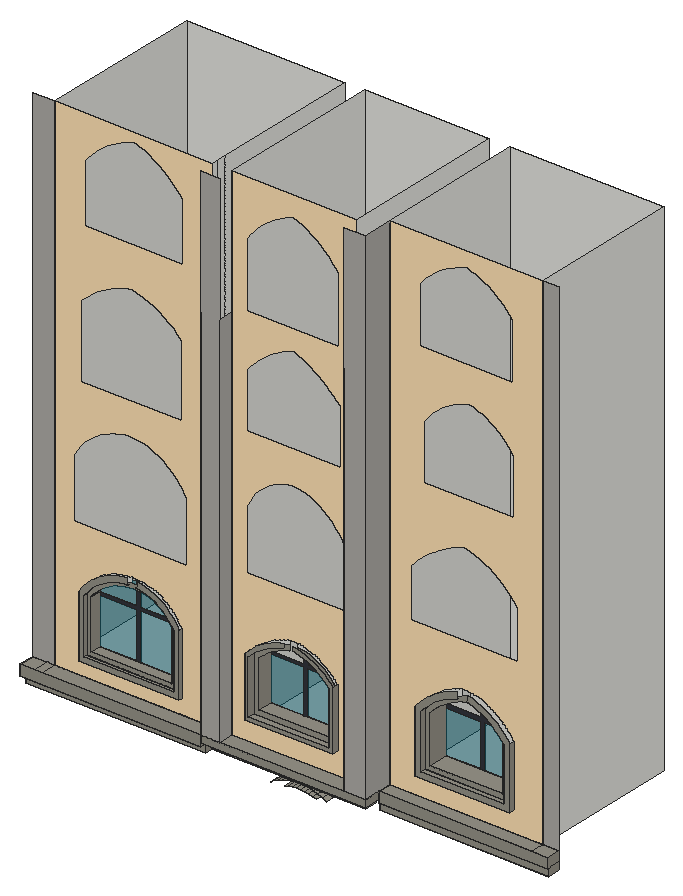
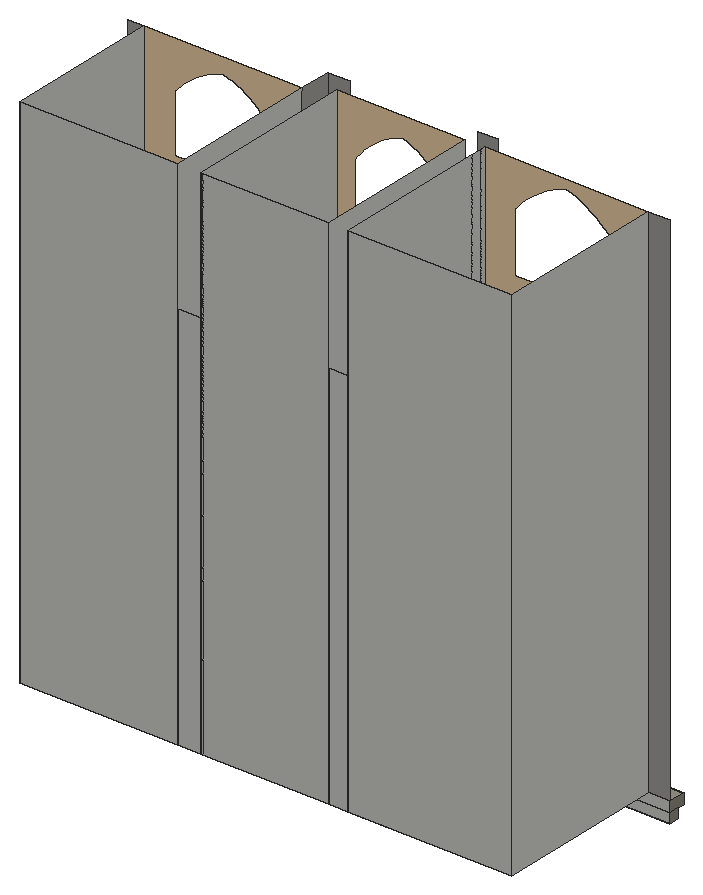
# SketchUp Ruby script. Lengths in inches.
U = 1.inch
M = Sketchup.active_model
def pt(a) = Geom::Point3d.new(a.map { |v| v * U })
def face(e, loops, mat)
  f = e.add_face(loops[0].map { |a| pt(a) })
  loops[1..].each { |l| e.add_face(l.map { |a| pt(a) }).erase! }
  f.material = f.back_material = mat if mat
  f
end
# faces: each face lists its corners as indices into pts; further lists are holes
def faces(e, pts, list, mat = nil) = list.each { |f| face(e, (f[0].is_a?(Array) ? f : [f]).map { |l| l.map { |i| pts[i] } }, mat) }
# xy, xz, yz: faces in a plane at the given z, y or x. An outline is a flat list of corners, or four numbers for a rectangle; further outlines are holes
def ring(l) = l.size == 4 ? [[l[0], l[1]], [l[2], l[1]], [l[2], l[3]], [l[0], l[3]]] : l.each_slice(2).to_a
def flat(e, list, mat, &to3) = list.each { |f| face(e, (f[0].is_a?(Array) ? f : [f]).map { |l| ring(l).map { |u, v| to3.(u, v) } }, mat) }
def xy(e, z, list, mat = nil) = flat(e, list, mat) { |x, y| [x, y, z] }
def xz(e, y, list, mat = nil) = flat(e, list, mat) { |x, z| [x, y, z] }
def yz(e, x, list, mat = nil) = flat(e, list, mat) { |y, z| [x, y, z] }
def lines(e, pts, list) = list.each { |a, b| e.add_line(pt(pts[a]), pt(pts[b])) }
# prism: a flat outline (further loops are holes) pulled along v
def prism(e, loops, v, mat = nil)
  f = face(e, loops, mat); d = Geom::Vector3d.new(v.map { |x| x * U })
  f.pushpull(f.normal.samedirection?(d) ? d.length : -d.length)
end
def box(e, o, s, mat = nil) = prism(e, [[o, [o[0] + s[0], o[1], o[2]], [o[0] + s[0], o[1] + s[1], o[2]], [o[0], o[1] + s[1], o[2]]]], [0, 0, s[2]], mat)
def at(x, y, z, deg = 0) = Geom::Transformation.translation(pt([x, y, z])) * Geom::Transformation.rotation(ORIGIN, Z_AXIS, deg.degrees)
def axes(o, x, y, z) = Geom::Transformation.new([*x, 0, *y, 0, *z, 0, *pt(o).to_a, 1])
def part(name) = M.definitions.add(name)
# library, detail: a bought-in or finely detailed component or shape, given as its bounding box
def library(name, o, s) = part(name).tap { |d| box(d.entities, o, s) }
def detail(e, o, s) = box(e.add_group.entities, o, s)
def put(e, d, t, mat = nil) = e.add_instance(d, t).tap { |i| i.material = mat if mat }
def group(e, t, mat = nil) = e.add_group.tap { |g| g.transformation = t; g.material = mat if mat }.entities
root = M.entities
M.materials.add("[Formica Beige]").color = [255, 225, 180]
M.materials.add("[Formica Graystone]").color = [149, 146, 135]
M.materials.add("[Formica Laminate Dark]").color = [50, 53, 60]
M.materials.add("[Terrazzo Tile Light]").color = [173, 171, 166]
M.materials.add("[Translucent Glass Tinted]").color = [4, 106, 127]
M.materials["[Translucent Glass Tinted]"].alpha = 0.48
xy(root,162.44,[[10.25,135.29,181.54,144.04]],"[Formica Graystone]")
xy(root,164.1875,[[338.35,146.55,499.12,158.3]],"[Formica Graystone]")
xy(root,167.08,[[186.17,137.18,186.17,148.61,199.67,148.61,199.67,158.3,317.75,158.3,317.75,148.61,332.68,148.61,332.68,137.18]],"[Formica Graystone]")
xy(root,171.09,[[10.25,135.29,181.54,144.04]])
xy(root,171.09,[[10.25,128.91,181.54,135.29]],"[Formica Graystone]")
xy(root,171.14,[[338.35,146.55,499.12,158.3]])
xy(root,171.14,[[338.35,145.11,499.12,146.55]],"[Formica Graystone]")
xy(root,174.01,[[186.17,137.18,186.17,148.61,199.67,148.61,199.67,158.3,317.75,158.3,317.75,148.61,332.68,148.61,332.68,137.18]])
xy(root,174.01,[[181.54,128.91,338.35,137.18],[181.54,137.18,186.17,148.61],[332.68,137.18,338.35,148.61]],"[Formica Graystone]")
xy(root,180.875,[[181.54,128.91,199.67,301.14],[317.75,128.91,338.35,158.3],[30.78,144.04,181.54,301.14],[199.67,144.04,317.75,158.3],[199.67,158.3,317.75,301.14],
  [317.75,158.3,338.35,301.14],[338.35,158.3,483.98,301.14]])
xy(root,180.875,[[10.25,128.91,24.51,144.04],[24.51,128.91,30.78,144.04],[30.78,128.91,181.54,144.04],[199.67,128.91,317.75,144.04],[338.35,145.11,483.98,158.3],
  [483.98,145.11,499.12,158.3]],"[Formica Graystone]")
xy(root,194.77,[[56.17,140.72,151.73,144.04]],"[Formica Graystone]")
xy(root,200.03,[[61.43,140.72,146.48,144.04]],"[Formica Graystone]")
xy(root,200.28,[[366.17,152.99,456.05,158.3]],"[Formica Graystone]")
xy(root,202.4375,[[216.67,137.35,300.3,144.04]],"[Formica Graystone]")
xy(root,203.83,[[65.22,144.04,142.68,154.66]],"[Formica Graystone]")
xy(root,205.7,[[371.6,152.99,450.625,158.3]],"[Formica Graystone]")
xy(root,206.125,[[220.36,137.35,296.61,144.04]],"[Formica Graystone]")
xy(root,210.3,[[376.19,158.3,446.03,177.43]],"[Formica Graystone]")
xy(root,210.91,[[225.15,144.04,291.83,158.22]],"[Formica Graystone]")
xz(root,128.91,[[10.25,171.09,181.54,180.875],[181.54,174.01,338.35,180.875]],"[Formica Graystone]")
xz(root,128.91,[[181.54,180.875,199.67,660.875],[317.75,180.875,338.35,660.875]],"[Terrazzo Tile Light]")
xz(root,135.29,[[10.25,162.44,181.54,171.09]],"[Formica Graystone]")
xz(root,137.18,[[186.17,167.08,332.68,174.01]],"[Formica Graystone]")
xz(root,137.35,[[216.67,202.4375,300.3,202.4375,300.3,258.75,297.68,261.875,294.86,264.8125,291.84,267.55,288.64,270.08,285.28,272.37,281.76,274.43,278.11,276.24,274.35,277.8,270.48,279.1,266.54,280.12,262.53,280.87,262.53,277.12,265.73,276.52,269.43,275.56,273.06,274.34,276.59,272.88,280.01,271.19,283.3,269.25,286.46,267.1,289.46,264.73,292.29,262.17,294.9375,259.41,296.61,257.41,296.61,206.125,220.36,206.125,220.36,257.22,222.06,258.93,224.9,261.5,227.88,263.91,230.98,266.16,234.2,268.25,237.52,270.16,240.9375,271.89,244.44,273.4375,248.03,274.8,251.68,275.97,254.54,276.72,254.54,280.53,250.64,279.51,246.81,278.28,243.04,276.85,239.36,275.22,235.76,273.4,232.27,271.4,228.89,269.21,225.63,266.84,222.51,264.3,219.52,261.6,216.67,258.75]],"[Formica Graystone]")
xz(root,140.72,[[56.17,194.77,151.73,194.77,151.73,253.84,149.35,258.08,146.5625,262.07,143.4,265.78,139.9,269.16,136.08,272.18,131.99,274.82,127.66,277.06,123.14,278.86,118.46,280.21,113.67,281.1,112.68,281.1875,112.68,276.05,111.06,276.05,112.96,275.88,117.24,275.09,121.43,273.875,125.48,272.26,129.35,270.27,133.02,267.9,136.43,265.2,139.57,262.17,142.4,258.86,144.89,255.28,146.48,252.46,146.48,200.03,61.43,200.03,61.43,252.15,63.1,254.5,65.9,257.84,68.95,260.96,72.23,263.83,75.73,266.4375,79.42,268.77,83.27,270.8,87.28,272.53,91.4,273.95,95.625,275.04,99.92,275.8,104.21,276.22,102.59,276.14,102.33,281.32,99.21,281.01,94.51,280.18,89.89,278.99,85.38,277.44,81,275.55,76.78,273.32,72.75,270.78,68.93,267.92,65.34,264.78,62,261.375,58.9375,257.72,56.17,253.84]],"[Formica Graystone]")
xz(root,144.04,[[10.25,162.44,181.54,171.09],[10.25,171.09,181.54,180.875],[56.17,194.77,56.17,253.84,58.9375,257.72,62,261.375,65.34,264.78,68.93,267.92,72.75,270.78,76.78,273.32,81,275.55,85.38,277.44,89.89,278.99,94.51,280.18,99.21,281.01,103.95,281.47,104.21,276.22,99.92,275.8,95.625,275.04,91.4,273.95,87.28,272.53,83.27,270.8,79.42,268.77,75.73,266.4375,72.23,263.83,68.95,260.96,65.9,257.84,63.1,254.5,61.43,252.15,61.43,200.03,146.48,200.03,146.48,252.46,144.89,255.28,142.4,258.86,139.57,262.17,136.43,265.2,133.02,267.9,129.35,270.27,125.48,272.26,121.43,273.875,117.24,275.09,112.96,275.88,111.06,276.05,111.06,281.33,113.67,281.1,118.46,280.21,123.14,278.86,127.66,277.06,131.99,274.82,136.08,272.18,139.9,269.16,143.4,265.78,146.5625,262.07,149.35,258.08,151.73,253.84,151.73,194.77],[216.67,202.4375,216.67,258.75,219.52,261.6,222.51,264.3,225.63,266.84,228.89,269.21,232.27,271.4,235.76,273.4,239.36,275.22,243.04,276.85,246.81,278.28,250.64,279.51,254.54,280.53,254.54,276.72,251.68,275.97,248.03,274.8,244.44,273.4375,240.9375,271.89,237.52,270.16,234.2,268.25,230.98,266.16,227.88,263.91,224.9,261.5,222.06,258.93,220.36,257.22,220.36,206.125,296.61,206.125,296.61,257.41,294.9375,259.41,292.29,262.17,289.46,264.73,286.46,267.1,283.3,269.25,280.01,271.19,276.59,272.88,273.06,274.34,269.43,275.56,265.73,276.52,262.53,277.12,262.53,280.87,266.54,280.12,270.48,279.1,274.35,277.8,278.11,276.24,281.76,274.43,285.28,272.37,288.64,270.08,291.84,267.55,294.86,264.8125,297.68,261.875,300.3,258.75,300.3,202.4375]])
xz(root,144.04,[[[30.78,180.875,181.54,660.875],[48.72,309.5625,48.72,366.1875,51.64,370.94,54.92,375.45,58.57,379.67,62.54,383.59,66.81,387.18,71.35,390.41,76.15,393.27,81.15,395.73,86.34,397.78,91.68,399.4,97.13,400.59,99.89,400.96,102.66,401.34,108.25,400.8125,113.78,399.8,119.2,398.3,124.46,396.33,129.53,393.91,134.375,391.05,138.94,387.77,143.21,384.11,147.13,380.09,150.69,375.74,153.85,371.09,156.59,366.1875,156.59,309.5625],[55.73,431.0625,55.73,499.48,59.68,503.46,63.87,507.2,68.28,510.68,72.89,513.875,77.69,516.79,82.66,519.4,87.78,521.7,93.03,523.68,98.39,525.34,103.85,526.66,109.32,525.375,114.7,523.75,119.96,521.79,125.1,519.51,130.08,516.9,134.89,513.99,139.5,510.79,143.91,507.3,148.09,503.55,152.02,499.53,152.02,431.0625],[56.17,194.77,56.17,253.84,58.9375,257.72,62,261.375,65.34,264.78,68.93,267.92,72.75,270.78,76.78,273.32,81,275.55,85.38,277.44,89.89,278.99,94.51,280.18,99.21,281.01,103.95,281.47,108.82,281.52,109.38,281.47,111.06,281.33,113.67,281.1,118.46,280.21,123.14,278.86,127.66,277.06,131.99,274.82,136.08,272.18,139.9,269.16,143.4,265.78,146.5625,262.07,149.35,258.08,151.73,253.84,151.73,194.77],[59.5,564.93,59.5,619.98,62.79,624.15,66.31,628.13,70.05,631.91,74,635.46,78.15,638.78,82.48,641.85,86.98,644.67,91.63,647.23,96.43,649.52,101.35,651.53,102.84,652.04,106.37,653.25,108.86,652.33,111.34,651.41,116.21,649.32,120.95,646.97,125.57,644.37,130.04,641.52,134.35,638.45,138.5,635.15,142.46,631.63,146.23,627.91,149.79,623.99,153.15,619.89,153.15,564.93]],[[199.67,180.875,317.75,660.875],[213.99,323.85,213.99,380.42,216.07,384.94,218.56,389.25,221.45,393.3125,224.71,397.08,228.31,400.52,232.22,403.6,236.4,406.31,240.82,408.6,245.4375,410.47,250.21,411.9,255.1,412.87,260.05,413.37,264.83,412.37,269.52,411,274.09,409.29,278.52,407.25,282.79,404.87,286.86,402.18,290.73,399.19,294.35,395.92,297.72,392.39,300.82,388.61,303.62,384.61,306.11,380.42,306.11,323.85],[213.99,546.83,213.99,608.29,216.9,612.46,220.05,616.45,223.44,620.24,227.05,623.83,230.86,627.2,234.87,630.33,239.06,633.22,243.41,635.85,247.91,638.22,252.55,640.31,257.3,642.13,262.125,640.46,266.83,638.48,271.4,636.1875,275.81,633.61,280.04,630.74,284.07,627.61,287.9,624.22,291.49,620.58,294.83,616.72,297.92,612.65,300.74,608.39,300.74,546.83],[213.87,444.43,213.87,496.8,216.84,500.3,219.97,503.65,223.25,506.87,226.66,509.93,230.21,512.84,233.89,515.59,237.68,518.16,241.59,520.57,245.6,522.8,249.71,524.84,253.91,526.7,258.18,528.37,262.4,526.6,266.55,524.66,270.62,522.55,274.59,520.28,278.48,517.86,282.26,515.28,285.93,512.55,289.49,509.67,292.9375,506.65,296.25,503.5,299.44,500.21,302.49,496.8,302.49,444.43],[216.67,202.4375,216.67,258.75,219.52,261.6,222.51,264.3,225.63,266.84,228.89,269.21,232.27,271.4,235.76,273.4,239.36,275.22,243.04,276.85,246.81,278.28,250.64,279.51,254.54,280.53,258.49,281.34,262.53,280.87,266.54,280.12,270.48,279.1,274.35,277.8,278.11,276.24,281.76,274.43,285.28,272.37,288.64,270.08,291.84,267.55,294.86,264.8125,297.68,261.875,300.3,258.75,300.3,202.4375]]],"[Formica Beige]")
xz(root,144.04,[[[61.43,200.03,146.48,200.03,146.48,252.46,144.89,255.28,142.4,258.86,139.57,262.17,136.43,265.2,133.02,267.9,129.35,270.27,125.48,272.26,121.43,273.875,117.24,275.09,112.96,275.88,111.06,276.05,109.15,276.22,104.21,276.22,99.92,275.8,95.625,275.04,91.4,273.95,87.28,272.53,83.27,270.8,79.42,268.77,75.73,266.4375,72.23,263.83,68.95,260.96,65.9,257.84,63.1,254.5,61.43,252.15],[65.22,203.83,65.22,250.9375,66.11,252.18,68.72,255.29,71.5625,258.2,74.62,260.875,77.88,263.31,81.32,265.48,84.92,267.375,88.65,268.99,92.49,270.31,96.43,271.33,100.4375,272.03,104.39,272.42,108.99,272.42,112.45,272.12,116.37,271.39,120.2,270.28,123.91,268.81,127.45,266.98,130.8,264.82,133.93,262.34,136.8,259.57,139.39,256.53,141.67,253.26,142.68,251.47,142.68,203.83]],[220.36,206.125,296.61,206.125,296.61,257.41,294.9375,259.41,292.29,262.17,289.46,264.73,286.46,267.1,283.3,269.25,280.01,271.19,276.59,272.88,273.06,274.34,269.43,275.56,265.73,276.52,262.53,277.12,262.53,272.25,264.69,271.85,268.07,270.97,271.38,269.86,274.61,268.53,277.73,266.97,280.74,265.21,283.63,263.24,286.37,261.08,288.95,258.74,291.37,256.22,291.83,255.67,291.83,210.91,225.15,210.91,225.15,255.25,225.36,255.46,228.02,257.86,230.79,260.12,233.69,262.22,236.69,264.16,239.79,265.95,242.99,267.57,246.26,269.01,249.6,270.28,253.01,271.37,254.54,271.77,254.54,276.72,251.68,275.97,248.03,274.8,244.44,273.4375,240.9375,271.89,237.52,270.16,234.2,268.25,230.98,266.16,227.88,263.91,224.9,261.5,222.06,258.93,220.36,257.22]],"[Formica Graystone]")
xz(root,144.04,[[10.25,180.875,30.78,660.875]],"[Terrazzo Tile Light]")
xz(root,145.11,[[338.35,171.14,499.12,180.875]],"[Formica Graystone]")
xz(root,146.55,[[338.35,164.1875,499.12,171.14]],"[Formica Graystone]")
xz(root,148.61,[[186.17,167.08,199.67,174.01],[317.75,167.08,332.68,174.01]])
xz(root,152.99,[[366.17,200.28,456.05,200.28,456.05,258.84,453.33,262.49,450.38,265.96,447.21,269.22,443.82,272.26,440.23,275.0625,436.47,277.625,432.55,279.93,428.47,281.96,424.28,283.72,419.97,285.2,416.39,286.16,416.39,280.76,415.58,280.76,418.38,280.01,422.35,278.65,426.21,277.03,429.96,275.16,433.57,273.04,437.03,270.68,440.33,268.1,443.45,265.3,446.37,262.3,449.09,259.11,450.625,257.05,450.625,205.7,371.6,205.7,371.6,256.87,373.14,258.7,376.02,261.77,379.0625,264.68,382.27,267.41,385.625,269.95,389.12,272.3,392.74,274.45,396.48,276.39,400.3125,278.12,404.24,279.63,406.74,280.43,405.62,280.43,405.62,285.77,402.44,284.75,398.22,283.13,394.11,281.28,390.1,279.19,386.22,276.89,382.47,274.37,378.87,271.64,375.43,268.71,372.16,265.6,369.07,262.3,366.17,258.84]],"[Formica Graystone]")
xz(root,154.66,[[100.4375,203.83,104.39,203.83,104.39,247.84,142.68,247.84,142.68,250.9375,104.39,250.9375,104.39,272.42,100.4375,272.03,100.4375,250.9375,65.22,250.9375,65.22,247.84,100.4375,247.84]],"[Formica Laminate Dark]")
xz(root,154.66,[[65.22,203.83,100.4375,247.84],[104.39,203.83,142.68,247.84],[65.22,250.9375,100.4375,250.9375,100.4375,272.03,96.43,271.33,92.49,270.31,88.65,268.99,84.92,267.375,81.32,265.48,77.88,263.31,74.62,260.875,71.5625,258.2,68.72,255.29,66.11,252.18],[104.39,250.9375,142.68,250.9375,142.68,251.47,141.67,253.26,139.39,256.53,136.8,259.57,133.93,262.34,130.8,264.82,127.45,266.98,123.91,268.81,120.2,270.28,116.37,271.39,112.45,272.12,108.99,272.42,104.39,272.42]],"[Translucent Glass Tinted]")
xz(root,158.22,[[256.47,210.91,260.2,210.91,260.2,252.26,291.83,252.26,291.83,255.25,260.2,255.25,260.2,272.49,258.86,272.77,256.47,272.28,256.47,255.25,225.15,255.25,225.15,252.26,256.47,252.26]],"[Formica Laminate Dark]")
xz(root,158.22,[[225.15,210.91,256.47,252.26],[260.2,210.91,291.83,252.26]],"[Translucent Glass Tinted]")
xz(root,158.3,[[338.35,164.1875,499.12,171.14],[199.67,167.08,317.75,174.01],[338.35,171.14,499.12,180.875],[199.67,174.01,317.75,180.875],[366.17,200.28,366.17,258.84,369.07,262.3,372.16,265.6,375.43,268.71,378.87,271.64,382.47,274.37,386.22,276.89,390.1,279.19,394.11,281.28,398.22,283.13,402.44,284.75,406.74,286.13,406.74,280.43,404.24,279.63,400.3125,278.12,396.48,276.39,392.74,274.45,389.12,272.3,385.625,269.95,382.27,267.41,379.0625,264.68,376.02,261.77,373.14,258.7,371.6,256.87,371.6,205.7,450.625,205.7,450.625,257.05,449.09,259.11,446.37,262.3,443.45,265.3,440.33,268.1,437.03,270.68,433.57,273.04,429.96,275.16,426.21,277.03,422.35,278.65,418.38,280.01,415.58,280.76,415.58,286.38,419.97,285.2,424.28,283.72,428.47,281.96,432.55,279.93,436.47,277.625,440.23,275.0625,443.82,272.26,447.21,269.22,450.38,265.96,453.33,262.49,456.05,258.84,456.05,200.28]])
xz(root,158.3,[[[338.35,180.875,483.98,660.875],[366.17,200.28,366.17,258.84,369.07,262.3,372.16,265.6,375.43,268.71,378.87,271.64,382.47,274.37,386.22,276.89,390.1,279.19,394.11,281.28,398.22,283.13,402.44,284.75,406.74,286.13,411.11,287.27,415.58,286.38,419.97,285.2,424.28,283.72,428.47,281.96,432.55,279.93,436.47,277.625,440.23,275.0625,443.82,272.26,447.21,269.22,450.38,265.96,453.33,262.49,456.05,258.84,456.05,200.28],[358.05,328.26,358.05,374.26,361.56,378.03,365.22,381.64,369.03,385.09,372.99,388.38,377.08,391.5,381.31,394.4375,385.65,397.19,390.1,399.77,394.66,402.14,399.32,404.33,404.07,406.31,408.9,408.09,413.875,406.64,418.76,404.93,423.55,402.94,428.22,400.69,432.76,398.19,437.15,395.44,441.39,392.45,445.45,389.23,449.33,385.79,453.01,382.14,456.48,378.3,459.74,374.26,459.74,328.26],[366.85,564.14,366.85,617.39,369.73,620.87,372.78,624.18,376.01,627.33,379.39,630.31,382.93,633.1,386.61,635.7,390.43,638.1,394.36,640.3,398.41,642.29,402.55,644.0625,406.79,645.61,411.09,646.9375,415.41,645.63,419.65,644.1,423.8,642.34,427.86,640.36,431.8,638.16,435.61,635.76,439.29,633.15,442.83,630.36,446.21,627.37,449.43,624.21,452.47,620.88,455.33,617.39,455.33,564.14],[370.76,449.51,370.76,500.95,373.34,504.58,376.14,508.06,379.15,511.35,382.35,514.45,385.74,517.35,389.31,520.03,393.03,522.49,396.9,524.71,400.9,526.69,405.01,528.42,409.22,529.89,413.52,531.1,417.87,530.02,422.13,528.65,426.29,526.99,430.34,525.06,434.24,522.86,437.99,520.4,441.56,517.7,444.94,514.76,448.12,511.6,451.07,508.24,453.8,504.68,456.27,500.95,456.27,449.51]]],"[Formica Beige]")
xz(root,158.3,[[[371.6,205.7,450.625,205.7,450.625,257.05,449.09,259.11,446.37,262.3,443.45,265.3,440.33,268.1,437.03,270.68,433.57,273.04,429.96,275.16,426.21,277.03,422.35,278.65,418.38,280.01,415.58,280.76,414.34,281.1,411.27,281.7,408.25,280.92,406.74,280.43,404.24,279.63,400.3125,278.12,396.48,276.39,392.74,274.45,389.12,272.3,385.625,269.95,382.27,267.41,379.0625,264.68,376.02,261.77,373.14,258.7,371.6,256.87],[376.19,210.3,376.19,255.2,376.57,255.66,379.28,258.54,382.14,261.27,385.15,263.83,388.3,266.21,391.58,268.42,394.97,270.4375,398.48,272.26,402.08,273.88,405.77,275.3,409.53,276.51,411.41,277,413.29,276.62,417.04,275.61,420.71,274.35,424.29,272.85,427.76,271.12,431.11,269.15,434.32,266.97,437.38,264.58,440.27,261.98,442.98,259.21,445.49,256.25,446.03,255.53,446.03,210.3]]],"[Formica Graystone]")
xz(root,158.3,[[483.98,180.875,499.12,660.875]],"[Terrazzo Tile Light]")
xz(root,177.43,[[409.53,210.3,413.29,210.3,413.29,251.17,446.03,251.17,446.03,255.2,413.29,255.2,413.29,276.62,411.41,277,409.53,276.51,409.53,255.2,376.19,255.2,376.19,251.17,409.53,251.17]],"[Formica Laminate Dark]")
xz(root,177.43,[[376.19,210.3,409.53,251.17],[413.29,210.3,446.03,251.17]],"[Translucent Glass Tinted]")
xz(root,301.14,[[30.78,180.875,181.54,660.875],[181.54,180.875,199.67,540.875],[199.67,180.875,315.73,660.875],[315.73,180.875,317.75,660.875],[317.75,180.875,338.35,540.875],
  [338.35,180.875,483.98,660.875]])
yz(root,10.25,[[135.29,162.44,144.04,171.09],[128.91,171.09,144.04,180.875]],"[Formica Graystone]")
yz(root,30.78,[[144.04,180.875,301.14,660.875]])
yz(root,56.17,[[140.72,194.77,144.04,253.84]],"[Formica Graystone]")
yz(root,61.43,[[140.72,200.03,144.04,252.15]],"[Formica Graystone]")
yz(root,65.22,[[144.04,203.83,154.66,250.9375]],"[Formica Graystone]")
yz(root,142.68,[[144.04,203.83,154.66,251.47]],"[Formica Graystone]")
yz(root,146.48,[[140.72,200.03,144.04,252.46]],"[Formica Graystone]")
yz(root,151.73,[[140.72,194.77,144.04,253.84]],"[Formica Graystone]")
yz(root,181.54,[[128.91,174.01,144.04,180.875],[144.04,174.01,148.61,180.875],[144.04,180.875,148.61,660.875],[148.61,180.875,158.3,660.875],[158.3,180.875,301.14,660.875]])
yz(root,181.54,[[135.29,162.44,144.04,171.09],[128.91,171.09,144.04,174.01]],"[Formica Graystone]")
yz(root,181.54,[[128.91,180.875,144.04,540.875]],"[Terrazzo Tile Light]")
yz(root,186.17,[[137.18,167.08,148.61,174.01]],"[Formica Graystone]")
yz(root,199.67,[[148.61,167.08,158.3,174.01],[148.61,174.01,158.3,180.875],[144.04,180.875,301.14,660.875]])
yz(root,199.67,[[128.91,180.875,144.04,540.875]],"[Terrazzo Tile Light]")
yz(root,216.67,[[137.35,202.4375,144.04,258.75]],"[Formica Graystone]")
yz(root,220.36,[[137.35,206.125,144.04,257.22]],"[Formica Graystone]")
yz(root,225.15,[[144.04,210.91,158.22,255.25]],"[Formica Graystone]")
yz(root,291.83,[[144.04,210.91,158.22,255.67]],"[Formica Graystone]")
yz(root,296.61,[[137.35,206.125,144.04,257.41]],"[Formica Graystone]")
yz(root,300.3,[[137.35,202.4375,144.04,258.75]],"[Formica Graystone]")
yz(root,317.75,[[148.61,167.08,158.3,174.01],[148.61,174.01,158.3,180.875],[144.04,180.875,301.14,660.875]])
yz(root,317.75,[[128.91,180.875,144.04,540.875]],"[Terrazzo Tile Light]")
yz(root,332.68,[[137.18,167.08,148.61,174.01]],"[Formica Graystone]")
yz(root,338.35,[[148.61,164.1875,158.3,171.14],[148.61,171.14,158.3,180.875],[145.11,174.01,148.61,180.875],[158.3,180.875,301.14,660.875]])
yz(root,338.35,[[146.55,164.1875,148.61,171.14],[145.11,171.14,148.61,174.01],[128.91,174.01,145.11,180.875]],"[Formica Graystone]")
yz(root,338.35,[[128.91,180.875,158.3,660.875]],"[Terrazzo Tile Light]")
yz(root,366.17,[[152.99,200.28,158.3,258.84]])
yz(root,371.6,[[152.99,205.7,158.3,256.87]],"[Formica Graystone]")
yz(root,376.19,[[158.3,210.3,177.43,255.2]],"[Formica Graystone]")
yz(root,446.03,[[158.3,210.3,177.43,255.53]],"[Formica Graystone]")
yz(root,450.625,[[152.99,205.7,158.3,257.05]],"[Formica Graystone]")
yz(root,456.05,[[152.99,200.28,158.3,258.84]],"[Formica Graystone]")
yz(root,483.98,[[158.3,180.875,301.14,660.875]])
yz(root,499.12,[[146.55,164.1875,158.3,171.14],[145.11,171.14,158.3,180.875]],"[Formica Graystone]")
p = [[234.81,158.3,151.28],[231.17,158.3,148.96],[231.17,150.74,148.96],[234.81,150.74,151.28],[270.68,158.3,150.24],[274.3,158.3,149.04],
  [274.3,150.74,149.04],[270.68,150.74,150.24],[244.39,158.3,149.82],[248.04,158.3,150.91],[248.04,150.74,150.91],[244.39,150.74,149.82],
  [266.97,158.3,151.15],[266.97,150.74,151.15],[283.86,158.3,150.39],[280.1,158.3,152.36],[280.1,150.74,152.36],[283.86,150.74,150.39],
  [251.78,158.3,151.64],[251.78,150.74,151.64],[263.19,158.3,151.76],[263.19,150.74,151.76],[238.64,158.3,153.25],[238.64,150.74,153.25],
  [255.57,158.3,152.03],[255.57,150.74,152.03],[259.4,158.3,152.06],[259.4,150.74,152.06],[276.18,158.3,154.02],[276.18,150.74,154.02],
  [242.64,158.3,154.85],[242.64,150.74,154.85],[272.15,158.3,155.36],[272.15,150.74,155.36],[246.77,158.3,156.08],[246.77,150.74,156.08],
  [268.02,158.3,156.37],[268.02,150.74,156.37],[250.99,158.3,156.91],[250.99,150.74,156.91],[263.83,158.3,157.04],[263.83,150.74,157.04],
  [255.28,158.3,157.35],[255.28,150.74,157.35],[259.59,158.3,157.38],[259.59,150.74,157.38],[66.11,144.04,252.18],[65.22,144.04,250.9375],
  [65.22,154.66,250.9375],[66.11,154.66,252.18],[142.68,144.04,251.47],[141.67,144.04,253.26],[141.67,154.66,253.26],[142.68,154.66,251.47],
  [61.43,144.04,252.15],[63.1,144.04,254.5],[63.1,140.72,254.5],[61.43,140.72,252.15],[68.72,144.04,255.29],[68.72,154.66,255.29],
  [144.89,144.04,255.28],[146.48,144.04,252.46],[146.48,140.72,252.46],[144.89,140.72,255.28],[139.39,144.04,256.53],[139.39,154.66,256.53]]
faces(root,p,[[0,1,2,3],[4,5,6,7],[8,9,10,11],[12,4,7,13],[14,15,16,17],[9,18,19,10],[20,12,13,21],[22,0,3,23],
  [18,24,25,19],[26,20,21,27],[24,26,27,25],[15,28,29,16],[30,22,23,31],[28,32,33,29],[34,30,31,35],[32,36,37,33],
  [38,34,35,39],[36,40,41,37],[42,38,39,43],[40,44,45,41],[44,42,43,45],[46,47,48,49],[50,51,52,53],[54,55,56,57],
  [58,46,49,59],[60,61,62,63],[51,64,65,52]],"[Formica Graystone]")
